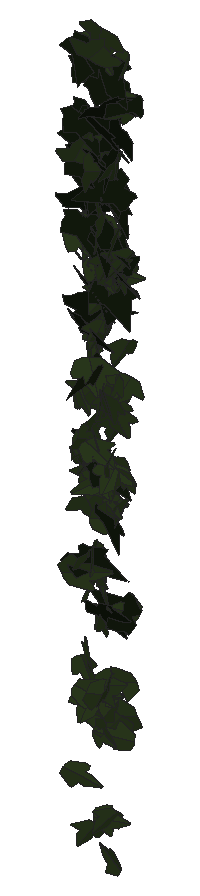
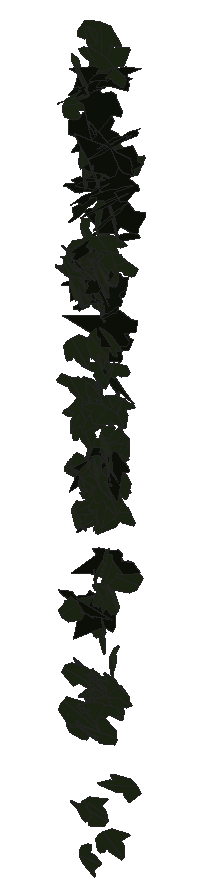
# SketchUp Ruby script. Lengths in inches.
U = 1.inch
M = Sketchup.active_model
def pt(a) = Geom::Point3d.new(a.map { |v| v * U })
def face(e, loops, mat)
  f = e.add_face(loops[0].map { |a| pt(a) })
  loops[1..].each { |l| e.add_face(l.map { |a| pt(a) }).erase! }
  f.material = f.back_material = mat if mat
  f
end
# faces: each face lists its corners as indices into pts; further lists are holes
def faces(e, pts, list, mat = nil) = list.each { |f| face(e, (f[0].is_a?(Array) ? f : [f]).map { |l| l.map { |i| pts[i] } }, mat) }
# xy, xz, yz: faces in a plane at the given z, y or x. An outline is a flat list of corners, or four numbers for a rectangle; further outlines are holes
def ring(l) = l.size == 4 ? [[l[0], l[1]], [l[2], l[1]], [l[2], l[3]], [l[0], l[3]]] : l.each_slice(2).to_a
def flat(e, list, mat, &to3) = list.each { |f| face(e, (f[0].is_a?(Array) ? f : [f]).map { |l| ring(l).map { |u, v| to3.(u, v) } }, mat) }
def xy(e, z, list, mat = nil) = flat(e, list, mat) { |x, y| [x, y, z] }
def xz(e, y, list, mat = nil) = flat(e, list, mat) { |x, z| [x, y, z] }
def yz(e, x, list, mat = nil) = flat(e, list, mat) { |y, z| [x, y, z] }
def lines(e, pts, list) = list.each { |a, b| e.add_line(pt(pts[a]), pt(pts[b])) }
# prism: a flat outline (further loops are holes) pulled along v
def prism(e, loops, v, mat = nil)
  f = face(e, loops, mat); d = Geom::Vector3d.new(v.map { |x| x * U })
  f.pushpull(f.normal.samedirection?(d) ? d.length : -d.length)
end
def box(e, o, s, mat = nil) = prism(e, [[o, [o[0] + s[0], o[1], o[2]], [o[0] + s[0], o[1] + s[1], o[2]], [o[0], o[1] + s[1], o[2]]]], [0, 0, s[2]], mat)
def at(x, y, z, deg = 0) = Geom::Transformation.translation(pt([x, y, z])) * Geom::Transformation.rotation(ORIGIN, Z_AXIS, deg.degrees)
def axes(o, x, y, z) = Geom::Transformation.new([*x, 0, *y, 0, *z, 0, *pt(o).to_a, 1])
def part(name) = M.definitions.add(name)
# library, detail: a bought-in or finely detailed component or shape, given as its bounding box
def library(name, o, s) = part(name).tap { |d| box(d.entities, o, s) }
def detail(e, o, s) = box(e.add_group.entities, o, s)
def put(e, d, t, mat = nil) = e.add_instance(d, t).tap { |i| i.material = mat if mat }
def group(e, t, mat = nil) = e.add_group.tap { |g| g.transformation = t; g.material = mat if mat }.entities
root = M.entities
M.materials.add("1026 AP 7946 SUNNY SIDE UP").color = [254, 231, 186]
M.materials.add("efeu1").color = [18, 25, 13]
M.materials.add("efeu2").color = [43, 57, 29]
c1 = part("ivyleaf_10")
p = [[0,0.5,-0.03],[-0.0625,2.02,-0.43],[-0.19,2.01,-0.46],[-0.54,1.05,-0.29],[-0.52,0.625,-0.18],[-0.83,0.76,-0.28],
  [-1.16,0.64,-0.33],[-1.15,0.33,-0.24],[-0.77,-0.39,0.02],[-0.3,-0.51,0.16],[0.04,-0.48,0.23],[-0.02,2.01,-0.4375],
  [-0.06,2.01,-0.43],[0.04,-0.49,0.23],[0.67,-0.49,0.14],[1.38,0.36,-0.2],[1.375,0.51,-0.24],[0.81,0.65,-0.19],
  [0.62,0.59,-0.15],[0.6,1.09,-0.28],[0.5,1.23,-0.31]]
faces(c1.entities,p,[[0,1,2,3,4,5,6,7,8,9,10],[11,12,0,13,14,15,16,17,18,19,20]],"efeu2")
c2 = part("ivyleaf_9")
p = [[1.54,2.16,1.25],[1.36,2.04,1.19],[-0.21,0.99,0.68],[-0.71,1.11,0.82],[-0.85,0.86,0.67],[-0.8,0.17,0.21],
  [-0.9,-0.01,0.1],[-0.67,-0.16,-0.02],[-0.08,-0.08,-0.05],[-0.03,-0.6,-0.4],[0.65,-0.88,-0.66],[0.83,-0.6,-0.49],
  [1.29,-0.42,-0.43],[1.8125,-0.07,-0.26],[1.21,0.44,0.15]]
faces(c2.entities,p,[[0,1,2,3,4,5,6,7,8,9,10,11,12,13,14]],"efeu1")
put(root,c1,axes([105.375,212.68,263.15],[-0.0201,-0.20981,0.14414],[0.05337,-0.14143,-0.2143],[0.39397,0.00846,0.03639]),"1026 AP 7946 SUNNY SIDE UP")
put(root,c2,axes([105.26,212.67,265.62],[-0.00257,-0.25191,0.01921],[-0.00005,-0.02008,-0.25964],[0.39736,-0.00163,0.00009]),"1026 AP 7946 SUNNY SIDE UP")
put(root,c1,axes([105.53,212.35,260.19],[-0.29267,-0.0712,0.1078],[-0.13209,-0.07064,-0.20308],[0.14957,-0.20171,0.03159]),"1026 AP 7946 SUNNY SIDE UP")
put(root,c1,axes([105.47,212.48,258.5],[-0.19203,-0.16937,0.05741],[-0.03711,-0.05277,-0.21511],[0.27838,-0.12387,0.01093]),"1026 AP 7946 SUNNY SIDE UP")
put(root,c1,axes([105.4375,212.54,258.81],[-0.03618,-0.1683,0.13894],[-0.00602,-0.13626,-0.17539],[0.34001,-0.02032,0.01168]),"1026 AP 7946 SUNNY SIDE UP")
put(root,c1,axes([105.35,212.2,264.93],[-0.23816,-0.21417,0.05044],[0.0352,0.0456,0.27038],[-0.34408,0.1529,-0.00725]),"1026 AP 7946 SUNNY SIDE UP")
put(root,c2,axes([105.31,212.68,264.1],[-0.04609,-0.19752,0.15159],[-0.00892,-0.14873,-0.20615],[0.38825,-0.02686,0.01326]),"1026 AP 7946 SUNNY SIDE UP")
put(root,c2,axes([105.5,212.43,259.12],[0.23251,0.03651,-0.19702],[-0.28896,-0.05395,-0.15713],[-0.1021,0.23582,-0.00396]),"1026 AP 7946 SUNNY SIDE UP")
put(root,c1,axes([105.22,212.48,254.54],[0.23827,-0.0354,0.14507],[0.21389,-0.03741,-0.16048],[0.08073,0.20359,-0.00299]),"1026 AP 7946 SUNNY SIDE UP")
put(root,c2,axes([105.39,212.53,267],[-0.18462,-0.22034,0.03499],[-0.00638,-0.03768,-0.25703],[0.35081,-0.11665,0.01374]),"1026 AP 7946 SUNNY SIDE UP")
put(root,c2,axes([105.26,212.36,265.67],[0.0537,-0.2376,-0.09022],[0.00308,0.08725,-0.24639],[0.39743,0.03143,0.0141]),"1026 AP 7946 SUNNY SIDE UP")
put(root,c1,axes([105.375,212.24,260.16],[-0.03657,0.21164,0.04728],[-0.00732,0.04445,-0.21908],[-0.34005,-0.02371,-0.00037]),"1026 AP 7946 SUNNY SIDE UP")
put(root,c2,axes([105.26,212.53,264.67],[-0.01445,-0.23399,-0.07711],[0.05989,0.07132,-0.23832],[0.38099,-0.02009,0.03454]),"1026 AP 7946 SUNNY SIDE UP")
put(root,c1,axes([105.26,212.43,258.81],[-0.27347,0.06232,-0.16233],[0.21754,-0.07901,-0.18955],[-0.15473,-0.22123,0.0204]),"1026 AP 7946 SUNNY SIDE UP")
put(root,c1,axes([105.18,212.44,263.18],[0.2653,0.08499,0.16639],[0.2479,0.04165,-0.19258],[-0.14324,0.22949,-0.0251]),"1026 AP 7946 SUNNY SIDE UP")
put(root,c1,axes([105.375,212.54,260.94],[-0.03523,0.21504,-0.05859],[0.01268,-0.05757,-0.22306],[-0.35002,-0.02373,-0.00219]),"1026 AP 7946 SUNNY SIDE UP")
put(root,c1,axes([105.45,212.28,259.09],[0.0131,-0.22839,-0.03888],[0.01371,0.03675,-0.235],[0.3634,0.00685,0.01027]),"1026 AP 7946 SUNNY SIDE UP")
put(root,c1,axes([105.47,212.35,264.11],[0.14163,-0.2185,-0.08118],[-0.03231,0.07536,-0.24285],[0.36314,0.09193,0.01005]),"1026 AP 7946 SUNNY SIDE UP")
put(root,c1,axes([105.2,212.21,252.45],[-0.10716,-0.03855,-0.1985],[0.30856,-0.01819,-0.06794],[-0.00728,-0.20337,0.04246]),"1026 AP 7946 SUNNY SIDE UP")
put(root,c2,axes([105.3125,212.32,263.87],[0.385,0.06454,0.08886],[-0.14127,0.00582,0.2594],[0.09261,-0.25941,0.02631]),"1026 AP 7946 SUNNY SIDE UP")
put(root,c2,axes([105.17,212.56,262.61],[0.26921,-0.17962,0.09351],[0.0759,-0.08042,-0.25533],[0.30796,0.17683,-0.01882]),"1026 AP 7946 SUNNY SIDE UP")
put(root,c1,axes([105.36,212.55,259.02],[0.22229,-0.1368,0.11749],[0.10373,-0.09609,-0.20217],[0.26097,0.15471,-0.01972]),"1026 AP 7946 SUNNY SIDE UP")
put(root,c2,axes([105.15,212.35,264.86],[0.37403,-0.02917,0.10778],[0.15678,-0.04226,-0.24553],[0.06837,0.25647,-0.02664]),"1026 AP 7946 SUNNY SIDE UP")
put(root,c1,axes([105.55,212.375,251.36],[-0.14524,-0.15934,0.10289],[-0.06196,-0.09343,-0.18993],[0.28991,-0.09979,0.01096]),"1026 AP 7946 SUNNY SIDE UP")
put(root,c1,axes([105.41,212.21,259.25],[0.03984,0.226,0.04176],[-0.00245,0.03966,-0.23397],[-0.36068,0.02469,0.00621]),"1026 AP 7946 SUNNY SIDE UP")
put(root,c1,axes([105.44,212.65,263.125],[0.14372,-0.20514,0.1002],[0.05327,-0.09262,-0.23182],[0.35379,0.09728,-0.0058]),"1026 AP 7946 SUNNY SIDE UP")
put(root,c2,axes([105.375,212.4375,265.16],[-0.23996,0.1208,0.18843],[0.20663,-0.12692,0.19931],[0.27474,0.20096,0.01468]),"1026 AP 7946 SUNNY SIDE UP")
put(root,c2,axes([105.29,212.46,265.11],[-0.14752,-0.00635,0.27471],[0.41742,0.02567,0.09698],[-0.04138,0.28154,-0.00099]),"1026 AP 7946 SUNNY SIDE UP")
put(root,c1,axes([105.51,212.43,258.22],[-0.21576,-0.17593,-0.04575],[0.06729,0.02145,-0.22878],[0.27686,-0.14231,0.01995]),"1026 AP 7946 SUNNY SIDE UP")
put(root,c1,axes([105.44,212.62,260.17],[-0.31222,-0.03741,-0.07802],[0.13246,-0.09385,-0.18083],[-0.00395,-0.19058,0.10293]),"1026 AP 7946 SUNNY SIDE UP")
put(root,c1,axes([105.63,212.14,254.87],[-0.01026,0.06969,-0.22526],[-0.11178,0.20779,0.07149],[0.34373,0.06965,0.01653]),"1026 AP 7946 SUNNY SIDE UP")
put(root,c1,axes([105.53,212.56,263.56],[0.32206,0.09606,-0.07942],[-0.10342,-0.04243,-0.23308],[-0.16439,0.21489,-0.00896]),"1026 AP 7946 SUNNY SIDE UP")
put(root,c1,axes([105.51,212.5,259.55],[0.07187,-0.1945,0.10648],[0.04318,-0.10084,-0.20639],[0.34445,0.05322,0.00366]),"1026 AP 7946 SUNNY SIDE UP")
put(root,c1,axes([105.49,212.09,259.35],[-0.04669,-0.14221,-0.2307],[0.10192,0.21378,-0.148],[0.40337,-0.07048,0.01069]),"1026 AP 7946 SUNNY SIDE UP")
put(root,c1,axes([105.52,212.49,261.65],[0.31813,-0.15231,-0.00725],[-0.0235,-0.00962,-0.26038],[0.23853,0.20218,-0.01599]),"1026 AP 7946 SUNNY SIDE UP")
put(root,c2,axes([105.47,212.72,264.32],[-0.12174,-0.23634,0.12039],[-0.02071,-0.11957,-0.25588],[0.415,-0.0753,0.02255]),"1026 AP 7946 SUNNY SIDE UP")
put(root,c1,axes([105.46,212.32,256.09],[0.09953,-0.21625,-0.00266],[0.01908,0.00215,0.23179],[-0.3395,-0.06328,0.01225]),"1026 AP 7946 SUNNY SIDE UP")
put(root,c2,axes([105.4,212.36,263.59],[-0.06037,-0.24842,-0.06961],[0.05148,0.06162,-0.25759],[0.40094,-0.04532,0.02259]),"1026 AP 7946 SUNNY SIDE UP")
put(root,c1,axes([105.3,212.1,256.53],[-0.1224,-0.04459,0.24996],[0.29029,0.15863,0.09188],[-0.25789,0.19973,-0.01521]),"1026 AP 7946 SUNNY SIDE UP")
put(root,c2,axes([105.23,212.38,261.72],[0.14757,0.0283,0.24911],[0.38256,-0.00966,-0.09623],[-0.00185,0.25905,-0.02927]),"1026 AP 7946 SUNNY SIDE UP")
put(root,c1,axes([105.54,212.25,256.9],[-0.10392,-0.18302,-0.11735],[0.0702,0.10383,-0.19977],[0.33074,-0.07954,0.00553]),"1026 AP 7946 SUNNY SIDE UP")
put(root,c1,axes([105.5,212.27,258],[-0.2619,-0.15002,-0.10714],[0.13523,0.05838,-0.23021],[0.25232,-0.18701,0.01218]),"1026 AP 7946 SUNNY SIDE UP")
put(root,c2,axes([105.27,212.39,261.38],[0.14041,-0.1187,0.20825],[0.18978,-0.16301,-0.15397],[0.31706,0.15013,-0.00006]),"1026 AP 7946 SUNNY SIDE UP")
put(root,c1,axes([105.69,212.21,259],[-0.07802,0.11519,0.18224],[-0.21009,0.12271,-0.12066],[-0.25586,-0.13588,0.0435]),"1026 AP 7946 SUNNY SIDE UP")
put(root,c1,axes([105.7,212.41,255.61],[-0.19828,0.11957,0.12986],[-0.18254,0.05679,-0.17575],[-0.20221,-0.16851,0.03132]),"1026 AP 7946 SUNNY SIDE UP")
put(root,c1,axes([105.61,212.37,259.35],[-0.12285,0.18574,0.09079],[-0.08198,0.07214,-0.20629],[-0.31196,-0.0921,0.01846]),"1026 AP 7946 SUNNY SIDE UP")
put(root,c1,axes([105.59,212.23,254.03],[0.26911,0.11238,-0.06518],[-0.06919,-0.04907,-0.21056],[-0.19115,0.17598,-0.01555]),"1026 AP 7946 SUNNY SIDE UP")
put(root,c2,axes([105.69,212.27,260.77],[-0.31522,0.11093,-0.13401],[0.15967,-0.08522,-0.23543],[-0.2172,-0.22363,0.02142]),"1026 AP 7946 SUNNY SIDE UP")
put(root,c1,axes([105.625,212.5625,258.96],[0.06324,-0.21242,0.00844],[-0.00052,-0.00963,-0.22276],[0.33433,0.04017,-0.00195]),"1026 AP 7946 SUNNY SIDE UP")
put(root,c1,axes([105.57,212.57,258.625],[0.32104,-0.01081,-0.0046],[-0.00857,-0.02008,-0.20971],[0.01623,0.20323,-0.01976]),"1026 AP 7946 SUNNY SIDE UP")
put(root,c1,axes([105.63,212.62,261.53],[0.00874,-0.21138,0.13157],[0.019,-0.12856,-0.21845],[0.38884,0.01103,0.00772]),"1026 AP 7946 SUNNY SIDE UP")
put(root,c1,axes([105.71,212.51,265.19],[-0.1587,-0.18635,0.13216],[-0.05631,-0.12671,-0.21759],[0.35222,-0.10422,0.02476]),"1026 AP 7946 SUNNY SIDE UP")
put(root,c1,axes([105.59,212.45,256.97],[-0.00315,0.17499,-0.17165],[-0.02559,-0.16734,-0.18075],[-0.38015,0.00982,0.01359]),"1026 AP 7946 SUNNY SIDE UP")
put(root,c2,axes([105.36,212.39,262.34],[0.21893,-0.19309,0.1144],[0.07904,-0.10166,-0.24522],[0.34209,0.14706,-0.01656]),"1026 AP 7946 SUNNY SIDE UP")
put(root,c1,axes([105.65,212.5,262.76],[0.14836,-0.22366,-0.00249],[-0.01659,-0.00321,-0.24984],[0.3513,0.09431,-0.01075]),"1026 AP 7946 SUNNY SIDE UP")
put(root,c1,axes([105.34,212.5625,267.125],[0.30432,0.0097,0.21414],[0.32669,-0.02352,-0.19834],[0.01672,0.283,-0.02216]),"1026 AP 7946 SUNNY SIDE UP")
put(root,c1,axes([105.6875,212.52,262.94],[0.25652,-0.14629,-0.08955],[-0.08871,0.0659,-0.22509],[0.25174,0.17229,0.01194]),"1026 AP 7946 SUNNY SIDE UP")
put(root,c1,axes([105.57,212.49,256.34],[-0.18693,0.13715,-0.10299],[0.09002,-0.0835,-0.18719],[-0.25199,-0.13157,0.00953]),"1026 AP 7946 SUNNY SIDE UP")
put(root,c1,axes([105.56,212.48,254.04],[0.2333,0.14213,0.0571],[0.07693,0.02772,-0.21105],[-0.22672,0.15566,-0.01286]),"1026 AP 7946 SUNNY SIDE UP")
put(root,c1,axes([105.71,212.34,264.16],[-0.06848,0.21423,0.10322],[-0.10475,0.08539,-0.22011],[-0.35598,-0.06634,0.04491]),"1026 AP 7946 SUNNY SIDE UP")
put(root,c2,axes([105.45,212.17,256.92],[0.02375,-0.02955,-0.24916],[0.16671,0.21879,-0.01945],[0.34467,-0.10379,0.02658]),"1026 AP 7946 SUNNY SIDE UP")
put(root,c1,axes([105.72,212.51,261.4],[-0.00238,-0.22772,0.01867],[-0.00236,-0.0194,-0.23471],[0.35936,-0.00164,-0.00142]),"1026 AP 7946 SUNNY SIDE UP")
put(root,c1,axes([105.72,212.41,261.54],[-0.0869,-0.20519,0.09957],[0.00599,-0.10149,-0.2177],[0.35738,-0.04819,0.02786]),"1026 AP 7946 SUNNY SIDE UP")
put(root,c2,axes([105.46,212.67,262.79],[0.08958,-0.17757,0.16144],[0.10131,-0.14455,-0.19248],[0.35943,0.085,0.01402]),"1026 AP 7946 SUNNY SIDE UP")
put(root,c1,axes([105.43,212.5,253.55],[0.00425,0.0034,0.21764],[0.31848,0.06003,-0.00331],[-0.09446,0.20255,-0.00138]),"1026 AP 7946 SUNNY SIDE UP")
put(root,c1,axes([105.82,212.31,258.5],[0.17884,0.06642,-0.20633],[-0.2443,-0.12821,-0.1352],[-0.22533,0.19173,-0.01717]),"1026 AP 7946 SUNNY SIDE UP")
put(root,c1,axes([105.68,212.04,264.83],[0.04086,-0.12009,-0.25026],[0.08824,0.24045,-0.11519],[0.41588,-0.03922,0.04903]),"1026 AP 7946 SUNNY SIDE UP")
put(root,c1,axes([105.5,212.16,254.21],[0.09966,0.08644,0.20899],[0.23675,0.13656,-0.10787],[-0.25236,0.16225,-0.01866]),"1026 AP 7946 SUNNY SIDE UP")
put(root,c1,axes([105.77,212.43,262.34],[0.22998,-0.17595,-0.04391],[-0.03225,0.03705,-0.23536],[0.28246,0.14748,0.00888]),"1026 AP 7946 SUNNY SIDE UP")
put(root,c1,axes([105.64,212.19,260.8],[0.28974,0.16701,0.04267],[0.06321,0.0158,-0.25563],[-0.2627,0.18799,-0.01444]),"1026 AP 7946 SUNNY SIDE UP")
put(root,c1,axes([105.86,212.24,267.58],[-0.41693,0.05119,0.05742],[-0.09298,-0.01506,-0.27705],[-0.07373,-0.27047,0.02465]),"1026 AP 7946 SUNNY SIDE UP")
put(root,c1,axes([105.68,212.24,267.0625],[-0.3616,-0.09516,0.11616],[0.1537,0.05947,0.25621],[-0.17465,0.24937,-0.01502]),"1026 AP 7946 SUNNY SIDE UP")
put(root,c1,axes([105.96,212.49,258.72],[-0.27734,-0.04643,-0.13916],[-0.21293,-0.01262,0.18692],[-0.07022,0.22165,-0.01714]),"1026 AP 7946 SUNNY SIDE UP")
put(root,c1,axes([105.65,212.54,256.47],[0.14254,-0.07463,0.18358],[0.19379,-0.12985,-0.12108],[0.23473,0.15252,-0.01151]),"1026 AP 7946 SUNNY SIDE UP")
put(root,c2,axes([105.59,212.3,265.67],[0.39316,-0.08727,-0.01077],[-0.02607,-0.01737,-0.272],[0.13563,0.24963,-0.02105]),"1026 AP 7946 SUNNY SIDE UP")
put(root,c2,axes([105.61,212.41,266.86],[-0.09418,-0.18915,-0.20665],[0.20553,0.16005,-0.1958],[0.38031,-0.13334,0.05464]),"1026 AP 7946 SUNNY SIDE UP")
put(root,c1,axes([105.93,212.37,262.33],[-0.17975,-0.17965,0.14681],[-0.07196,-0.1393,-0.21799],[0.35433,-0.11943,0.0302]),"1026 AP 7946 SUNNY SIDE UP")
put(root,c1,axes([105.5625,212.41,262.74],[0.21774,0.002,0.21676],[0.32483,-0.04907,-0.13988],[0.06276,0.24705,-0.02803]),"1026 AP 7946 SUNNY SIDE UP")
put(root,c1,axes([105.69,212.36,258.14],[-0.26255,-0.02371,-0.14058],[0.21757,-0.03014,-0.16937],[-0.00155,-0.21344,0.03825]),"1026 AP 7946 SUNNY SIDE UP")
put(root,c1,axes([105.77,212.22,257.74],[0.0013,0.0372,0.23328],[0.02067,0.22585,-0.03698],[-0.35991,0.01311,-0.00128]),"1026 AP 7946 SUNNY SIDE UP")
put(root,c1,axes([105.68,212.18,259.17],[0.17466,0.12079,0.14626],[0.16043,0.09796,-0.16834],[-0.24432,0.15068,-0.00598]),"1026 AP 7946 SUNNY SIDE UP")
put(root,c1,axes([105.75,212.35,263.63],[0.0973,-0.14672,0.21239],[0.16814,-0.17814,-0.16405],[0.36179,0.12225,0.01912]),"1026 AP 7946 SUNNY SIDE UP")
put(root,c1,axes([105.84,212.47,259.99],[-0.32513,-0.07982,-0.05935],[0.09309,0.00493,-0.2277],[0.12314,-0.21447,0.01542]),"1026 AP 7946 SUNNY SIDE UP")
put(root,c2,axes([105.75,212.58,264.46],[0.00166,-0.24162,-0.01156],[0.00271,0.00986,-0.24886],[0.38023,0.00098,0.00182]),"1026 AP 7946 SUNNY SIDE UP")
put(root,c1,axes([106.07,212.35,250.78],[-0.08136,0.03243,-0.21231],[-0.21915,0.15287,0.06167],[0.24448,0.14783,-0.01537]),"1026 AP 7946 SUNNY SIDE UP")
put(root,c1,axes([105.76,212.33,260.25],[0.1543,-0.11193,0.17462],[0.16377,-0.13471,-0.15398],[0.27518,0.14293,-0.00628]),"1026 AP 7946 SUNNY SIDE UP")
put(root,c1,axes([105.75,212.34,258.14],[-0.12116,-0.09781,-0.2041],[0.22076,0.13958,-0.12679],[0.26724,-0.15964,0.0122]),"1026 AP 7946 SUNNY SIDE UP")
put(root,c2,axes([105.76,212.3,255.9],[0.37468,0.03688,-0.03718],[-0.05048,-0.02882,-0.24741],[-0.06382,0.2393,-0.02262]),"1026 AP 7946 SUNNY SIDE UP")
put(root,c1,axes([105.76,212.12,254.26],[-0.06044,-0.07181,-0.22603],[0.22003,0.16914,-0.08145],[0.28795,-0.14432,0.0148]),"1026 AP 7946 SUNNY SIDE UP")
put(root,c1,axes([105.91,212.53,260.47],[0.28865,-0.11965,-0.04142],[-0.04712,0.02639,-0.22551],[0.19245,0.18592,0.00691]),"1026 AP 7946 SUNNY SIDE UP")
put(root,c2,axes([105.93,212.1,266.18],[0.13381,0.26154,0.03043],[0.0311,0.02304,-0.28295],[-0.41243,0.08659,-0.01146]),"1026 AP 7946 SUNNY SIDE UP")
put(root,c1,axes([105.91,212.23,260.27],[-0.10514,0.21497,0.05921],[-0.04178,0.05059,-0.2314],[-0.34689,-0.07125,0.00992]),"1026 AP 7946 SUNNY SIDE UP")
put(root,c1,axes([105.97,212.55,259.64],[-0.11329,-0.19326,0.0453],[-0.01466,-0.0446,-0.21263],[0.31169,-0.07234,0.00646]),"1026 AP 7946 SUNNY SIDE UP")
put(root,c2,axes([105.8,212.51,263.42],[0.09076,-0.19986,-0.14589],[-0.06001,0.13519,-0.21351],[0.3794,0.06919,0.00113]),"1026 AP 7946 SUNNY SIDE UP")
put(root,c1,axes([106.07,212.46,253.68],[-0.27052,-0.03899,0.10929],[-0.14636,-0.0614,-0.17875],[0.10138,-0.19269,0.03356]),"1026 AP 7946 SUNNY SIDE UP")
put(root,c2,axes([105.87,212.53,265.11],[-0.21131,0.04574,-0.22076],[0.30515,-0.09253,-0.14609],[-0.16083,-0.23565,0.01287]),"1026 AP 7946 SUNNY SIDE UP")
put(root,c2,axes([105.79,212.36,263.25],[0.03263,-0.21405,0.1235],[0.00055,-0.1215,-0.22202],[0.3867,0.01823,-0.0101]),"1026 AP 7946 SUNNY SIDE UP")
put(root,c2,axes([106.14,212.45,264.46],[-0.31485,-0.07554,0.13818],[-0.18399,-0.06938,-0.21991],[0.15818,-0.23105,0.01925]),"1026 AP 7946 SUNNY SIDE UP")
put(root,c2,axes([105.79,212.29,266.58],[0.14187,-0.16808,-0.1814],[-0.0409,0.17907,-0.1898],[0.37948,0.08214,0.04736]),"1026 AP 7946 SUNNY SIDE UP")
put(root,c1,axes([105.99,212.2,254.38],[0.00025,-0.17583,-0.16116],[-0.00299,0.15543,-0.18023],[0.36901,0.00138,-0.00135]),"1026 AP 7946 SUNNY SIDE UP")
put(root,c1,axes([106.04,212.3,251.8],[-0.10518,-0.14141,0.13461],[-0.06157,-0.12631,-0.16123],[0.2973,-0.07619,0.01424]),"1026 AP 7946 SUNNY SIDE UP")
put(root,c1,axes([105.72,212.32,253.41],[0.03532,0.01873,0.2156],[0.31188,-0.07105,-0.0158],[0.10855,0.19802,-0.02475]),"1026 AP 7946 SUNNY SIDE UP")
put(root,c2,axes([105.81,212.38,263.53],[0.17968,-0.20009,-0.09253],[-0.0534,0.08262,-0.23664],[0.33997,0.11873,0.01174]),"1026 AP 7946 SUNNY SIDE UP")
put(root,c2,axes([105.87,212.3,258.83],[0.03882,-0.15958,-0.19101],[-0.04526,0.18225,-0.16528],[0.38089,0.03792,-0.00017]),"1026 AP 7946 SUNNY SIDE UP")
put(root,c1,axes([106.03,212.26,263.09],[-0.11176,-0.22527,0.07286],[-0.01289,-0.0728,-0.24338],[0.37165,-0.07027,0.01347]),"1026 AP 7946 SUNNY SIDE UP")
put(root,c1,axes([106.07,212.15,258.94],[0.03458,0.03896,0.22239],[-0.18067,0.1866,-0.02157],[-0.29341,-0.11031,0.03949]),"1026 AP 7946 SUNNY SIDE UP")
put(root,c1,axes([105.93,212.27,253.86],[0.04796,0.07215,-0.21],[0.09761,0.19471,0.08154],[0.32634,-0.06884,0.00647]),"1026 AP 7946 SUNNY SIDE UP")
put(root,c1,axes([106.14,212.58,262.87],[-0.09118,-0.04993,-0.23013],[-0.24149,-0.16199,0.07753],[-0.2663,0.164,0.00849]),"1026 AP 7946 SUNNY SIDE UP")
put(root,c1,axes([105.8,212.22,258.62],[0.10717,0.01082,-0.20974],[0.24769,0.13359,0.0624],[0.20368,-0.16815,0.03447]),"1026 AP 7946 SUNNY SIDE UP")
put(root,c2,axes([105.88,212.45,262.15],[-0.08199,-0.19148,0.16569],[0.0523,-0.1692,-0.19609],[0.39082,-0.01753,0.061]),"1026 AP 7946 SUNNY SIDE UP")
put(root,c2,axes([105.85,212.42,257.76],[0.07219,-0.22439,0.11355],[0.02482,-0.11054,-0.23652],[0.39321,0.04817,-0.00592]),"1026 AP 7946 SUNNY SIDE UP")
put(root,c1,axes([106.08,212.4,258.71],[-0.34263,0.00976,0.02611],[-0.04108,-0.02115,-0.22367],[-0.01133,-0.21834,0.02154]),"1026 AP 7946 SUNNY SIDE UP")
put(root,c1,axes([105.99,212.49,260.03],[-0.11255,-0.18064,-0.12807],[0.09555,0.10819,-0.19901],[0.33035,-0.09284,0.01393]),"1026 AP 7946 SUNNY SIDE UP")
put(root,c2,axes([106.18,212.36,265.69],[0.18189,-0.02357,-0.25252],[-0.38637,0.00437,-0.11993],[0.02206,0.27089,-0.01844]),"1026 AP 7946 SUNNY SIDE UP")
put(root,c1,axes([106.29,212.51,253.8],[-0.14897,0.01241,0.22159],[-0.33539,-0.03802,-0.09478],[0.04702,-0.23187,0.026]),"1026 AP 7946 SUNNY SIDE UP")
put(root,c2,axes([106.18,212.38,262.81],[-0.31241,0.12403,-0.10207],[-0.11558,0.07007,0.24091],[0.22201,0.211,-0.01821]),"1026 AP 7946 SUNNY SIDE UP")
put(root,c1,axes([106.03,212.65,257.93],[0.05073,-0.19262,0.08919],[0.03766,-0.08479,-0.20149],[0.33063,0.03921,0.00927]),"1026 AP 7946 SUNNY SIDE UP")
put(root,c2,axes([106.35,212.41,255.9],[-0.26663,-0.02889,-0.18391],[-0.27795,-0.02407,0.17701],[-0.05878,0.24492,-0.00283]),"1026 AP 7946 SUNNY SIDE UP")
put(root,c1,axes([106.08,212.31,265],[-0.00582,-0.25106,-0.11975],[0.00539,0.11478,-0.25799],[0.43405,-0.00479,0.0016]),"1026 AP 7946 SUNNY SIDE UP")
put(root,c2,axes([105.75,212.39,262.92],[0.25985,-0.15765,0.13975],[0.12454,-0.11373,-0.23469],[0.30339,0.18172,-0.02336]),"1026 AP 7946 SUNNY SIDE UP")
put(root,c1,axes([106.04,212.2,260.26],[-0.31194,0.0979,-0.01525],[0.00856,-0.02355,-0.22723],[-0.15559,-0.19758,0.01807]),"1026 AP 7946 SUNNY SIDE UP")
put(root,c1,axes([106.09,212.43,262.62],[-0.10689,-0.21902,0.04918],[-0.0068,-0.04989,-0.2363],[0.35283,-0.06732,0.01034]),"1026 AP 7946 SUNNY SIDE UP")
put(root,c2,axes([105.87,212.58,264.125],[0.0833,-0.23385,0.07221],[0.02069,-0.07024,-0.24741],[0.38392,0.05453,-0.00234]),"1026 AP 7946 SUNNY SIDE UP")
put(root,c1,axes([106.08,212.41,262.72],[0.27515,-0.12421,-0.09861],[-0.06519,0.10064,-0.21361],[0.23711,0.17181,0.0557]),"1026 AP 7946 SUNNY SIDE UP")
put(root,c1,axes([106.05,212.61,266.9375],[0.23394,-0.21771,0.01493],[-0.00351,-0.02055,-0.27142],[0.3432,0.14819,-0.01295]),"1026 AP 7946 SUNNY SIDE UP")
put(root,c1,axes([105.8,212.31,251.66],[0.06373,-0.04528,-0.19985],[0.30228,-0.04202,0.05131],[-0.08059,-0.19342,0.03439]),"1026 AP 7946 SUNNY SIDE UP")
put(root,c1,axes([105.8,212.3125,254.33],[0.15267,-0.10772,-0.20168],[0.2746,-0.09553,0.14327],[-0.21783,-0.19593,0.03926]),"1026 AP 7946 SUNNY SIDE UP")
put(root,c1,axes([106.01,212.41,259.83],[-0.30784,-0.07223,-0.07667],[0.11693,0.0118,-0.21444],[0.113,-0.20897,0.01302]),"1026 AP 7946 SUNNY SIDE UP")
put(root,c1,axes([106.07,212.32,258.78],[0.27166,0.12496,-0.08927],[-0.09134,-0.06812,-0.21914],[-0.22167,0.18122,-0.0191]),"1026 AP 7946 SUNNY SIDE UP")
put(root,c1,axes([106.28,212.46,254.51],[0.14472,-0.03419,-0.19906],[-0.3005,0.03186,-0.0995],[0.06867,0.21146,-0.0159]),"1026 AP 7946 SUNNY SIDE UP")
put(root,c1,axes([106.29,212.38,253.39],[-0.00057,0.03993,0.20937],[-0.27938,-0.10408,0.02015],[0.1667,-0.1743,0.03449]),"1026 AP 7946 SUNNY SIDE UP")
put(root,c1,axes([106.14,212.56,261.24],[-0.10606,-0.19759,0.08486],[-0.02099,-0.08349,-0.21514],[0.33664,-0.06745,0.01332]),"1026 AP 7946 SUNNY SIDE UP")
put(root,c1,axes([105.78,212.45,262.62],[0.07341,-0.06316,-0.24697],[0.38927,0.01082,0.04686],[-0.00174,-0.24364,0.06458]),"1026 AP 7946 SUNNY SIDE UP")
put(root,c1,axes([106.04,212.4,263.5],[0.15629,-0.19344,0.1202],[0.07686,-0.10727,-0.22462],[0.34772,0.11066,-0.00438]),"1026 AP 7946 SUNNY SIDE UP")
put(root,c1,axes([106.17,212.44,262.92],[-0.20512,-0.21394,0.06891],[-0.0318,-0.06725,-0.25793],[0.3516,-0.13089,0.01688]),"1026 AP 7946 SUNNY SIDE UP")
put(root,c1,axes([106.14,212.46,258.66],[0.30632,-0.05121,-0.0769],[-0.09403,0.05931,-0.20312],[0.10636,0.1999,0.04191]),"1026 AP 7946 SUNNY SIDE UP")
put(root,c1,axes([106.125,212.59,262.52],[0.07372,-0.22959,0.02825],[0.0018,-0.02908,-0.24152],[0.36381,0.04667,-0.00453]),"1026 AP 7946 SUNNY SIDE UP")
put(root,c1,axes([106.12,212.48,262.58],[-0.03129,-0.21231,0.11909],[0.03319,-0.11827,-0.21846],[0.37958,-0.00716,0.02891]),"1026 AP 7946 SUNNY SIDE UP")
put(root,c1,axes([106.15,212.57,260.49],[0.3437,-0.00949,-0.04599],[-0.0703,-0.00186,-0.22537],[0.01404,0.22307,-0.00253]),"1026 AP 7946 SUNNY SIDE UP")
put(root,c2,axes([106.14,212.64,266.28],[-0.20054,-0.17313,0.14369],[-0.02915,-0.15302,-0.21255],[0.34935,-0.11216,0.06475]),"1026 AP 7946 SUNNY SIDE UP")
put(root,c2,axes([106.02,212.3125,262.46],[-0.07342,-0.20312,-0.13215],[0.08278,0.11765,-0.2129],[0.36757,-0.06706,0.02155]),"1026 AP 7946 SUNNY SIDE UP")
put(root,c1,axes([106.07,212.32,258.63],[0.22048,-0.11261,0.1066],[0.10525,-0.08199,-0.18471],[0.21698,0.1542,-0.01872]),"1026 AP 7946 SUNNY SIDE UP")
put(root,c1,axes([106.21,212.59,266.08],[-0.07231,-0.00755,0.26068],[0.0031,-0.25723,-0.00904],[0.39812,0.00063,0.04742]),"1026 AP 7946 SUNNY SIDE UP")
put(root,c1,axes([106.2,212.5,263.07],[0.00309,-0.16388,0.18698],[0.00336,-0.18242,-0.1699],[0.38558,0.0029,-0.00002]),"1026 AP 7946 SUNNY SIDE UP")
put(root,c1,axes([106.23,212.625,255.82],[0.01202,0.11244,0.21255],[-0.03538,-0.20449,0.11482],[0.36688,-0.0234,0.00411]),"1026 AP 7946 SUNNY SIDE UP")
